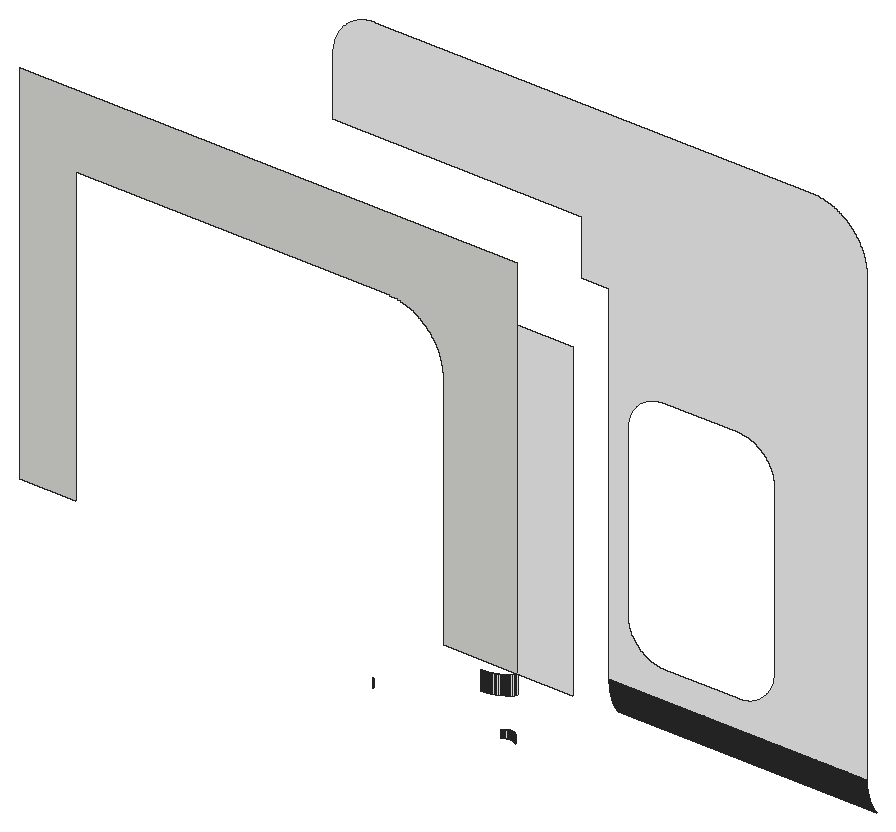
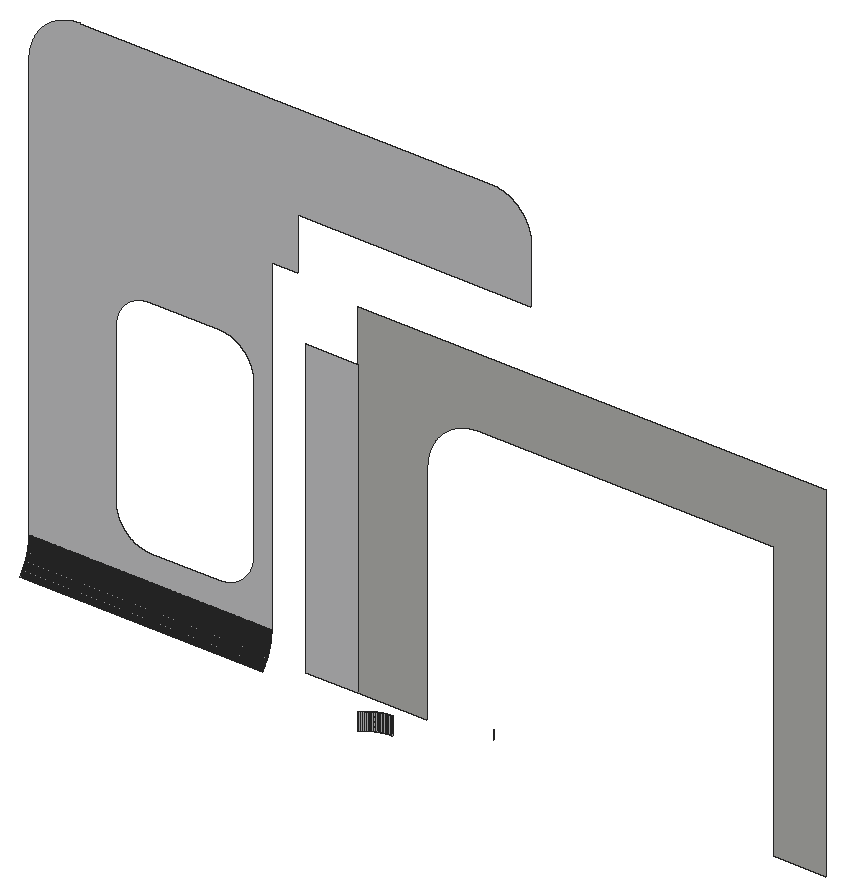
# SketchUp Ruby script. Lengths in inches.
U = 1.inch
M = Sketchup.active_model
def pt(a) = Geom::Point3d.new(a.map { |v| v * U })
def face(e, loops, mat)
  f = e.add_face(loops[0].map { |a| pt(a) })
  loops[1..].each { |l| e.add_face(l.map { |a| pt(a) }).erase! }
  f.material = f.back_material = mat if mat
  f
end
# faces: each face lists its corners as indices into pts; further lists are holes
def faces(e, pts, list, mat = nil) = list.each { |f| face(e, (f[0].is_a?(Array) ? f : [f]).map { |l| l.map { |i| pts[i] } }, mat) }
# xy, xz, yz: faces in a plane at the given z, y or x. An outline is a flat list of corners, or four numbers for a rectangle; further outlines are holes
def ring(l) = l.size == 4 ? [[l[0], l[1]], [l[2], l[1]], [l[2], l[3]], [l[0], l[3]]] : l.each_slice(2).to_a
def flat(e, list, mat, &to3) = list.each { |f| face(e, (f[0].is_a?(Array) ? f : [f]).map { |l| ring(l).map { |u, v| to3.(u, v) } }, mat) }
def xy(e, z, list, mat = nil) = flat(e, list, mat) { |x, y| [x, y, z] }
def xz(e, y, list, mat = nil) = flat(e, list, mat) { |x, z| [x, y, z] }
def yz(e, x, list, mat = nil) = flat(e, list, mat) { |y, z| [x, y, z] }
def lines(e, pts, list) = list.each { |a, b| e.add_line(pt(pts[a]), pt(pts[b])) }
# prism: a flat outline (further loops are holes) pulled along v
def prism(e, loops, v, mat = nil)
  f = face(e, loops, mat); d = Geom::Vector3d.new(v.map { |x| x * U })
  f.pushpull(f.normal.samedirection?(d) ? d.length : -d.length)
end
def box(e, o, s, mat = nil) = prism(e, [[o, [o[0] + s[0], o[1], o[2]], [o[0] + s[0], o[1] + s[1], o[2]], [o[0], o[1] + s[1], o[2]]]], [0, 0, s[2]], mat)
def at(x, y, z, deg = 0) = Geom::Transformation.translation(pt([x, y, z])) * Geom::Transformation.rotation(ORIGIN, Z_AXIS, deg.degrees)
def axes(o, x, y, z) = Geom::Transformation.new([*x, 0, *y, 0, *z, 0, *pt(o).to_a, 1])
def part(name) = M.definitions.add(name)
# library, detail: a bought-in or finely detailed component or shape, given as its bounding box
def library(name, o, s) = part(name).tap { |d| box(d.entities, o, s) }
def detail(e, o, s) = box(e.add_group.entities, o, s)
def put(e, d, t, mat = nil) = e.add_instance(d, t).tap { |i| i.material = mat if mat }
def group(e, t, mat = nil) = e.add_group.tap { |g| g.transformation = t; g.material = mat if mat }.entities
root = M.entities
M.materials.add("[Quartz Light Grey]").color = [251, 251, 252]
xz(root,256,[[207.84,117,207.92,119.5],[207.92,117,208,119.5],[208,117,208.08,119.5],[208.08,117,208.16,119.5]],"[Quartz Light Grey]")
xz(root,271,[[36,126,54,126,54,222,156.4,222,156.61,221.99,157.21,221.96,157.41,221.94,157.61,221.93,157.81,221.91,158.02,221.89,158.22,221.86,158.42,221.84,159.02,221.75,159.21,221.71,160.01,221.55,160.2,221.5,160.4,221.45,160.59,221.4,160.79,221.35,160.98,221.3,161.18,221.24,161.37,221.18,161.5625,221.12,161.75,221.06,161.95,220.99,162.14,220.92,162.32,220.85,162.7,220.71,162.89,220.63,163.07,220.55,163.26,220.47,163.44,220.39,163.63,220.3,163.81,220.22,164.35,219.95,164.71,219.75,164.88,219.66,165.06,219.55,165.4,219.35,165.58,219.24,165.92,219.02,166.08,218.91,166.25,218.8,166.42,218.68,166.58,218.5625,166.74,218.44,166.9,218.32,167.0625,218.2,167.22,218.07,167.38,217.95,167.54,217.82,167.69,217.6875,167.84,217.56,167.99,217.42,168.14,217.29,168.29,217.15,168.4375,217.01,168.58,216.87,168.73,216.73,168.87,216.58,169.01,216.4375,169.15,216.29,169.29,216.14,169.42,215.99,169.56,215.84,169.6875,215.69,169.82,215.54,169.95,215.38,170.07,215.22,170.2,215.0625,170.32,214.9,170.44,214.74,170.5625,214.58,170.68,214.42,170.8,214.25,170.91,214.08,171.02,213.92,171.24,213.58,171.35,213.4,171.55,213.06,171.66,212.88,171.75,212.71,171.95,212.35,172.22,211.81,172.3,211.63,172.39,211.44,172.47,211.26,172.55,211.07,172.63,210.89,172.71,210.7,172.85,210.32,172.92,210.14,172.99,209.95,173.06,209.75,173.12,209.5625,173.18,209.37,173.24,209.18,173.3,208.98,173.35,208.79,173.4,208.59,173.45,208.4,173.5,208.2,173.55,208.01,173.71,207.21,173.75,207.02,173.84,206.42,173.86,206.22,173.89,206.02,173.91,205.81,173.93,205.61,173.94,205.41,173.96,205.21,173.99,204.61,174,204.4,174,126,198,126,198,246,36,246]])
xz(root,271,[[186,117,186.16,123],[186.16,117,186.3125,123],[198,126,216,228],[228,134.77,312,135],[[228,135,312,135,312,282.24,311.99,282.47,311.99,282.71,311.98,282.94,311.96,283.18,311.94,283.41,311.92,283.65,311.9,283.88,311.875,284.12,311.85,284.35,311.8125,284.58,311.78,284.82,311.7,285.28,311.65,285.51,311.61,285.74,311.56,285.97,311.5,286.2,311.45,286.43,311.39,286.66,311.32,286.89,311.26,287.11,311.19,287.34,311.12,287.5625,311.04,287.79,310.97,288.01,310.89,288.23,310.8,288.45,310.72,288.67,310.54,289.11,310.44,289.32,310.35,289.54,310.25,289.75,310.14,289.96,310.04,290.17,309.82,290.59,309.7,290.8,309.59,291,309.35,291.4,309.22,291.61,309.1,291.8,308.97,292,308.83,292.2,308.7,292.39,308.5625,292.58,308.42,292.77,308.28,292.96,308.14,293.14,307.99,293.33,307.84,293.51,307.6875,293.69,307.53,293.87,307.375,294.04,307.22,294.22,307.06,294.39,306.89,294.56,306.73,294.73,306.56,294.89,306.39,295.06,306.22,295.22,306.04,295.375,305.87,295.53,305.69,295.6875,305.51,295.84,305.33,295.99,305.14,296.14,304.96,296.28,304.77,296.42,304.58,296.5625,304.39,296.7,304.2,296.83,304,296.97,303.8,297.1,303.61,297.22,303.4,297.35,303,297.59,302.8,297.7,302.59,297.82,302.17,298.04,301.96,298.14,301.75,298.25,301.54,298.35,301.32,298.44,301.11,298.54,300.67,298.72,300.45,298.8,300.23,298.89,300.01,298.97,299.79,299.04,299.5625,299.12,299.34,299.19,299.11,299.26,298.89,299.32,298.66,299.39,298.43,299.45,298.2,299.5,297.97,299.56,297.74,299.61,297.51,299.65,297.28,299.7,296.82,299.78,296.58,299.8125,296.35,299.85,296.12,299.875,295.88,299.9,295.65,299.92,295.41,299.94,295.18,299.96,294.94,299.98,294.71,299.99,294.47,299.99,294.24,300,151.63,300,151.27,299.98,151.08,299.97,150.9,299.96,150.54,299.92,150.35,299.9,149.99,299.86,149.45,299.77,148.55,299.57,148.2,299.47,148.02,299.42,147.85,299.37,147.67,299.31,147.5,299.26,147.33,299.2,147.15,299.13,146.98,299.07,146.8125,299,146.64,298.93,146.47,298.86,146.31,298.79,146.14,298.71,145.97,298.64,145.81,298.56,145.64,298.47,145.48,298.39,145.16,298.21,145,298.125,144.84,298.03,144.69,297.9375,144.53,297.84,144.22,297.64,144.07,297.54,143.92,297.43,143.77,297.33,143.48,297.11,143.33,296.99,143.19,296.88,143.05,296.76,142.91,296.65,142.77,296.53,142.63,296.4,142.5,296.28,142.36,296.16,141.84,295.64,141.72,295.5,141.6,295.37,141.47,295.23,141.35,295.09,141.24,294.95,141.12,294.81,141.01,294.67,140.89,294.52,140.67,294.23,140.57,294.08,140.46,293.93,140.36,293.78,140.16,293.47,140.0625,293.31,139.97,293.16,139.875,293,139.79,292.84,139.61,292.52,139.53,292.36,139.44,292.19,139.36,292.03,139.29,291.86,139.21,291.69,139.14,291.53,139.07,291.36,139,291.1875,138.93,291.02,138.87,290.85,138.8,290.67,138.74,290.5,138.69,290.33,138.63,290.15,138.58,289.98,138.53,289.8,138.43,289.45,138.23,288.55,138.14,288.01,138.1,287.65,138.08,287.46,138.04,287.1,138.03,286.92,138.02,286.73,138,286.37,138,267,219,267,219,249,228,249],[245.84,144,245.6875,144.01,245.53,144.01,245.37,144.02,245.22,144.03,244.9,144.05,244.75,144.07,244.59,144.08,244.43,144.1,244.28,144.125,244.12,144.15,243.97,144.17,243.8125,144.2,243.66,144.23,243.51,144.26,243.35,144.3,243.2,144.33,243.05,144.37,242.89,144.41,242.74,144.45,242.59,144.5,242.44,144.54,241.99,144.69,241.85,144.74,241.55,144.86,241.41,144.91,241.26,144.98,240.98,145.1,240.83,145.17,240.41,145.38,240.27,145.46,240.14,145.53,240,145.61,239.86,145.6875,239.73,145.77,239.6,145.85,239.46,145.9375,239.33,146.02,239.07,146.2,238.95,146.29,238.82,146.39,238.7,146.48,238.57,146.58,238.45,146.68,238.33,146.77,238.09,146.98,237.97,147.08,237.85,147.1875,237.74,147.3,237.52,147.52,237.4,147.63,237.3,147.74,237.1875,147.86,237.08,147.97,236.98,148.09,236.77,148.33,236.67,148.45,236.58,148.57,236.48,148.7,236.39,148.82,236.29,148.95,236.2,149.07,236.02,149.33,235.9375,149.47,235.85,149.6,235.77,149.73,235.6875,149.87,235.61,150,235.53,150.14,235.45,150.27,235.17,150.83,235.1,150.98,235.04,151.12,234.97,151.26,234.91,151.41,234.85,151.55,234.8,151.7,234.74,151.85,234.6875,151.99,234.64,152.14,234.49,152.59,234.41,152.89,234.37,153.05,234.33,153.2,234.3,153.35,234.26,153.51,234.23,153.66,234.2,153.8125,234.17,153.97,234.15,154.12,234.125,154.28,234.1,154.43,234.08,154.59,234.07,154.75,234.05,154.9,234.03,155.22,234.02,155.37,234.01,155.53,234,155.6875,234,210.3125,234.01,210.47,234.02,210.63,234.03,210.78,234.05,211.1,234.07,211.25,234.08,211.41,234.1,211.57,234.125,211.72,234.15,211.88,234.17,212.03,234.2,212.1875,234.23,212.34,234.26,212.49,234.3,212.65,234.33,212.8,234.37,212.95,234.41,213.11,234.49,213.41,234.64,213.86,234.6875,214.01,234.74,214.15,234.8,214.3,234.85,214.45,234.91,214.59,234.97,214.74,235.04,214.88,235.1,215.02,235.17,215.17,235.45,215.73,235.53,215.86,235.61,216,235.6875,216.14,235.77,216.27,235.85,216.4,235.9375,216.54,236.02,216.67,236.2,216.93,236.29,217.05,236.38,217.18,236.48,217.31,236.58,217.43,236.67,217.55,236.77,217.67,236.98,217.91,237.08,218.03,237.1875,218.15,237.3,218.26,237.4,218.375,237.51,218.49,237.625,218.6,237.74,218.7,237.85,218.8125,237.97,218.92,238.09,219.02,238.33,219.23,238.45,219.33,238.57,219.42,238.69,219.52,238.82,219.62,238.95,219.71,239.07,219.8,239.33,219.98,239.46,220.0625,239.6,220.15,239.73,220.23,239.86,220.3125,240,220.39,240.14,220.47,240.27,220.55,240.83,220.83,240.98,220.9,241.12,220.96,241.26,221.03,241.41,221.09,241.55,221.15,241.7,221.2,241.85,221.26,241.99,221.3125,242.14,221.36,242.59,221.51,242.89,221.59,243.05,221.63,243.2,221.67,243.35,221.7,243.51,221.74,243.66,221.77,243.8125,221.8,243.97,221.83,244.12,221.85,244.28,221.875,244.43,221.9,244.59,221.92,244.75,221.93,244.9,221.95,245.22,221.97,245.37,221.98,245.53,221.99,245.6875,222,270.3125,222,270.47,221.99,270.63,221.98,270.78,221.97,271.1,221.95,271.25,221.93,271.41,221.92,271.57,221.9,271.72,221.875,271.88,221.85,272.03,221.83,272.1875,221.8,272.34,221.77,272.49,221.74,272.65,221.7,272.8,221.67,272.95,221.63,273.11,221.59,273.41,221.51,273.86,221.36,274.01,221.3125,274.15,221.26,274.3,221.2,274.45,221.15,274.59,221.09,274.74,221.03,274.88,220.96,275.02,220.9,275.17,220.83,275.73,220.55,275.86,220.47,276,220.39,276.14,220.3125,276.27,220.23,276.4,220.15,276.54,220.0625,276.67,219.98,276.93,219.8,277.05,219.71,277.18,219.62,277.31,219.52,277.43,219.42,277.55,219.33,277.67,219.23,277.91,219.02,278.03,218.92,278.15,218.8125,278.26,218.7,278.375,218.6,278.49,218.49,278.6,218.375,278.7,218.26,278.8125,218.15,278.92,218.03,279.02,217.91,279.23,217.67,279.33,217.55,279.42,217.43,279.52,217.31,279.62,217.18,279.71,217.05,279.8,216.93,279.98,216.67,280.0625,216.54,280.15,216.4,280.23,216.27,280.3125,216.14,280.39,216,280.47,215.86,280.55,215.73,280.83,215.17,280.9,215.02,280.96,214.88,281.03,214.74,281.09,214.59,281.15,214.45,281.2,214.3,281.26,214.15,281.3125,214.01,281.36,213.86,281.51,213.41,281.59,213.11,281.63,212.95,281.67,212.8,281.7,212.65,281.74,212.49,281.77,212.34,281.8,212.1875,281.83,212.03,281.85,211.88,281.875,211.72,281.9,211.57,281.92,211.41,281.93,211.25,281.95,211.1,281.97,210.78,281.98,210.63,281.99,210.47,282,210.3125,282,155.6875,281.99,155.53,281.98,155.37,281.97,155.22,281.95,154.9,281.93,154.75,281.92,154.59,281.9,154.43,281.875,154.28,281.85,154.12,281.83,153.97,281.8,153.8125,281.77,153.66,281.74,153.51,281.7,153.35,281.67,153.2,281.63,153.05,281.59,152.89,281.51,152.59,281.36,152.14,281.3125,151.99,281.26,151.85,281.2,151.7,281.15,151.55,281.09,151.41,281.03,151.26,280.96,151.12,280.9,150.98,280.83,150.83,280.55,150.27,280.47,150.14,280.39,150,280.3125,149.87,280.23,149.73,280.15,149.6,280.0625,149.47,279.98,149.33,279.8,149.07,279.71,148.95,279.61,148.82,279.52,148.7,279.42,148.57,279.33,148.45,279.23,148.33,279.02,148.09,278.92,147.97,278.8125,147.86,278.7,147.74,278.6,147.63,278.48,147.52,278.26,147.3,278.15,147.1875,278.03,147.08,277.91,146.98,277.67,146.77,277.55,146.68,277.43,146.58,277.3,146.48,277.18,146.39,277.05,146.29,276.93,146.2,276.67,146.02,276.54,145.9375,276.4,145.85,276.27,145.77,276.14,145.6875,276,145.61,275.86,145.53,275.73,145.46,275.59,145.38,275.17,145.17,275.02,145.1,274.74,144.98,274.59,144.91,274.45,144.86,274.15,144.74,274.01,144.69,273.56,144.54,273.41,144.5,273.26,144.45,273.11,144.41,272.95,144.37,272.8,144.33,272.65,144.3,272.49,144.26,272.34,144.23,272.1875,144.2,272.03,144.17,271.88,144.15,271.72,144.125,271.57,144.1,271.41,144.08,271.25,144.07,271.1,144.05,270.78,144.03,270.63,144.02,270.47,144.01,270.3125,144.01,270.16,144]]],"[Quartz Light Grey]")
xz(root,271.01,[[228,134.29,312,134.53]],"[Quartz Light Grey]")
p = [[164,254.89,117],[164.05,254.83,117],[164.05,254.83,119.5],[164,254.89,119.5],[163.9,255.01,117],[163.95,254.95,117],
  [163.95,254.95,119.5],[163.9,255.01,119.5],[205.67,254.89,117],[205.72,254.95,117],[205.72,254.95,119.5],[205.67,254.89,119.5],
  [205.77,255.01,117],[205.77,255.01,119.5],[210.23,255.01,117],[210.28,254.95,117],[210.28,254.95,119.5],[210.23,255.01,119.5],
  [210.33,254.89,117],[210.33,254.89,119.5],[163.84,255.07,117],[163.84,255.07,119.5],[205.82,255.07,117],[205.82,255.07,119.5],
  [210.18,255.07,117],[210.18,255.07,119.5],[163.73,255.18,117],[163.79,255.12,117],[163.79,255.12,119.5],[163.73,255.18,119.5],
  [205.88,255.12,117],[205.88,255.12,119.5],[205.93,255.18,117],[205.93,255.18,119.5],[210.07,255.18,117],[210.12,255.12,117],
  [210.12,255.12,119.5],[210.07,255.18,119.5],[163.62,255.28,117],[163.67,255.23,117],[163.67,255.23,119.5],[163.62,255.28,119.5],
  [205.99,255.23,117],[205.99,255.23,119.5],[206.05,255.28,117],[206.05,255.28,119.5],[209.95,255.28,117],[210.01,255.23,117],
  [210.01,255.23,119.5],[209.95,255.28,119.5],[163.49,255.38,117],[163.55,255.33,117],[163.55,255.33,119.5],[163.49,255.38,119.5],
  [206.11,255.33,117],[206.11,255.33,119.5],[206.17,255.38,117],[206.17,255.38,119.5],[209.83,255.38,117],[209.89,255.33,117],
  [209.89,255.33,119.5],[209.83,255.38,119.5],[163.37,255.47,117],[163.43,255.43,117],[163.43,255.43,119.5],[163.37,255.47,119.5],
  [206.24,255.43,117],[206.24,255.43,119.5],[206.3,255.47,117],[206.3,255.47,119.5],[209.7,255.47,117],[209.76,255.43,117],
  [209.76,255.43,119.5],[209.7,255.47,119.5],[163.3,255.52,117],[163.3,255.52,119.5],[206.37,255.52,117],[206.37,255.52,119.5],
  [206.43,255.56,117],[206.43,255.56,119.5],[209.57,255.56,117],[209.63,255.52,117],[209.63,255.52,119.5],[209.57,255.56,119.5],
  [206.5,255.6,117],[206.5,255.6,119.5],[206.57,255.64,117],[206.57,255.64,119.5],[206.64,255.67,117],[206.64,255.67,119.5],
  [209.36,255.67,117],[209.43,255.64,117],[209.43,255.64,119.5],[209.36,255.67,119.5],[209.5,255.6,117],[209.5,255.6,119.5],
  [206.71,255.71,117],[206.71,255.71,119.5],[206.78,255.74,117],[206.78,255.74,119.5],[206.85,255.77,117],[206.85,255.77,119.5],
  [209.15,255.77,117],[209.22,255.74,117],[209.22,255.74,119.5],[209.15,255.77,119.5],[209.29,255.71,117],[209.29,255.71,119.5],
  [206.92,255.8,117],[206.92,255.8,119.5],[207,255.83,117],[207,255.83,119.5],[207.07,255.85,117],[207.07,255.85,119.5],
  [208.93,255.85,117],[209,255.83,117],[209,255.83,119.5],[208.93,255.85,119.5],[209.08,255.8,117],[209.08,255.8,119.5],
  [207.15,255.875,117],[207.15,255.875,119.5],[207.22,255.9,117],[207.22,255.9,119.5],[207.3,255.92,117],[207.3,255.92,119.5],
  [207.375,255.93,117],[207.375,255.93,119.5],[207.45,255.95,117],[207.45,255.95,119.5],[207.53,255.96,117],[207.53,255.96,119.5],
  [208.47,255.96,117],[208.55,255.95,117],[208.55,255.95,119.5],[208.47,255.96,119.5],[208.625,255.93,117],[208.625,255.93,119.5],
  [208.7,255.92,117],[208.7,255.92,119.5],[208.78,255.9,117],[208.78,255.9,119.5],[208.85,255.875,117],[208.85,255.875,119.5],
  [207.61,255.97,117],[207.61,255.97,119.5],[207.6875,255.98,117],[207.6875,255.98,119.5],[207.76,255.99,117],[207.76,255.99,119.5],
  [207.84,256,117],[207.84,256,119.5],[208.16,256,117],[208.24,255.99,117],[208.24,255.99,119.5],[208.16,256,119.5],
  [208.3125,255.98,117],[208.3125,255.98,119.5],[208.39,255.97,117],[208.39,255.97,119.5],[186.47,271.01,117],[186.3125,271,117],
  [186.3125,271,123],[186.47,271.01,123],[186.63,271.02,117],[186.63,271.02,123],[186.78,271.03,117],[186.78,271.03,123],
  [186.94,271.04,117],[186.94,271.04,123],[187.1,271.05,117],[187.1,271.05,123],[187.25,271.07,117],[187.25,271.07,123],
  [187.41,271.08,117],[187.41,271.08,123],[187.57,271.1,117],[187.57,271.1,123],[187.72,271.125,117],[187.72,271.125,123],
  [187.88,271.15,117],[187.88,271.15,123],[188.03,271.17,117],[188.03,271.17,123],[188.1875,271.2,117],[188.1875,271.2,123],
  [188.34,271.23,117],[188.34,271.23,123],[188.49,271.26,117],[188.49,271.26,123],[188.65,271.3,117],[188.65,271.3,123],
  [188.8,271.33,117],[188.8,271.33,123],[188.95,271.37,117],[188.95,271.37,123],[189.11,271.41,117],[189.11,271.41,123],
  [189.26,271.45,117],[189.26,271.45,123],[189.41,271.49,117],[189.41,271.49,123],[189.56,271.54,117],[189.56,271.54,123],
  [189.71,271.59,117],[189.71,271.59,123],[189.86,271.64,117],[189.86,271.64,123],[190.01,271.6875,117],[190.01,271.6875,123],
  [190.15,271.74,117],[190.15,271.74,123],[190.3,271.8,117],[190.3,271.8,123],[190.45,271.85,117],[190.45,271.85,123],
  [190.59,271.91,117],[190.59,271.91,123],[190.74,271.97,117],[190.74,271.97,123],[190.88,272.04,117],[190.88,272.04,123],
  [191.02,272.1,117],[191.02,272.1,123],[191.17,272.17,117],[191.17,272.17,123],[191.31,272.24,117],[191.31,272.24,123],
  [191.45,272.31,117],[191.45,272.31,123],[191.59,272.38,117],[191.59,272.38,123],[191.73,272.45,117],[191.73,272.45,123],
  [191.86,272.53,117],[191.86,272.53,123],[192,272.61,117],[192,272.61,123],[192.14,272.6875,117],[192.14,272.6875,123],
  [192.27,272.77,117],[192.27,272.77,123],[192.4,272.85,117],[192.4,272.85,123],[192.54,272.9375,117],[192.54,272.9375,123],
  [192.67,273.02,117],[192.67,273.02,123],[192.8,273.11,117],[192.8,273.11,123],[192.93,273.2,117],[192.93,273.2,123],
  [193.05,273.29,117],[193.05,273.29,123],[193.18,273.38,117],[193.18,273.38,123],[193.31,273.48,117],[193.31,273.48,123],
  [193.43,273.58,117],[193.43,273.58,123],[193.55,273.67,117],[193.55,273.67,123],[193.67,273.77,117],[193.67,273.77,123],
  [193.79,273.875,117],[193.79,273.875,123],[193.91,273.98,117],[193.91,273.98,123],[194.03,274.08,117],[194.03,274.08,123],
  [194.15,274.1875,117],[194.15,274.1875,123],[194.26,274.3,117],[194.26,274.3,123],[194.375,274.4,117],[194.375,274.4,123],
  [194.49,274.51,117],[194.49,274.51,123],[194.6,274.625,117],[194.6,274.625,123],[194.7,274.74,117],[194.7,274.74,123],
  [194.8125,274.85,117],[194.8125,274.85,123],[194.92,274.97,117],[194.92,274.97,123],[312,274.86,123.86],[312,274.72,124.04],
  [228,274.72,124.04],[228,274.86,123.86],[312,274.58,124.23],[228,274.58,124.23],[312,274.4375,124.42],[228,274.4375,124.42],
  [312,274.3,124.61],[228,274.3,124.61],[312,274.17,124.81],[228,274.17,124.81],[312,274.03,125],[228,274.03,125],
  [312,273.9,125.2],[228,273.9,125.2],[312,273.78,125.4],[228,273.78,125.4],[312,273.65,125.6],[228,273.65,125.6],
  [312,273.53,125.8],[228,273.53,125.8],[312,273.41,126],[228,273.41,126],[312,273.3,126.21],[228,273.3,126.21],
  [312,273.18,126.41],[228,273.18,126.41],[312,273.07,126.62],[228,273.07,126.62],[312,272.96,126.83],[228,272.96,126.83],
  [312,272.86,127.04],[228,272.86,127.04],[312,272.75,127.25],[228,272.75,127.25],[312,272.65,127.46],[228,272.65,127.46],
  [312,272.56,127.68],[228,272.56,127.68],[312,272.46,127.9],[228,272.46,127.9],[312,272.37,128.11],[228,272.37,128.11],
  [312,272.28,128.33],[228,272.28,128.33],[312,272.2,128.55],[228,272.2,128.55],[312,272.11,128.77],[228,272.11,128.77],
  [312,272.03,128.99],[228,272.03,128.99],[312,271.96,129.22],[228,271.96,129.22],[312,271.88,129.4375],[228,271.88,129.4375],
  [312,271.81,129.66],[228,271.81,129.66],[312,271.74,129.89],[228,271.74,129.89],[312,271.68,130.12],[228,271.68,130.12],
  [312,271.61,130.34],[228,271.61,130.34],[312,271.55,130.57],[228,271.55,130.57],[312,271.5,130.8],[228,271.5,130.8],
  [312,271.44,131.03],[228,271.44,131.03],[312,271.39,131.26],[228,271.39,131.26],[312,271.35,131.49],[228,271.35,131.49],
  [312,271.3,131.72],[228,271.3,131.72],[312,271.26,131.95],[228,271.26,131.95],[312,271.22,132.19],[228,271.22,132.19],
  [312,271.1875,132.42],[228,271.1875,132.42],[312,271.15,132.65],[228,271.15,132.65],[312,271.125,132.89],[228,271.125,132.89],
  [312,271.1,133.12],[228,271.1,133.12],[312,271.08,133.35],[228,271.08,133.35],[312,271.06,133.59],[228,271.06,133.59],
  [312,271.04,133.82],[228,271.04,133.82],[312,271.02,134.06],[228,271.02,134.06],[312,271.01,134.29],[228,271.01,134.29],
  [312,271.01,134.53],[312,271,134.77],[228,271,134.77],[228,271.01,134.53]]
faces(root,p,[[0,1,2,3],[4,5,6,7],[5,0,3,6],[8,9,10,11],[9,12,13,10],[14,15,16,17],[15,18,19,16],[20,4,7,21],
  [12,22,23,13],[24,14,17,25],[26,27,28,29],[27,20,21,28],[22,30,31,23],[30,32,33,31],[34,35,36,37],[35,24,25,36],
  [38,39,40,41],[39,26,29,40],[32,42,43,33],[42,44,45,43],[46,47,48,49],[47,34,37,48],[50,51,52,53],[51,38,41,52],
  [44,54,55,45],[54,56,57,55],[58,59,60,61],[59,46,49,60],[62,63,64,65],[63,50,53,64],[56,66,67,57],[66,68,69,67],
  [70,71,72,73],[71,58,61,72],[74,62,65,75],[68,76,77,69],[76,78,79,77],[80,81,82,83],[81,70,73,82],[78,84,85,79],
  [84,86,87,85],[86,88,89,87],[90,91,92,93],[91,94,95,92],[94,80,83,95],[88,96,97,89],[96,98,99,97],[98,100,101,99],
  [102,103,104,105],[103,106,107,104],[106,90,93,107],[100,108,109,101],[108,110,111,109],[110,112,113,111],[114,115,116,117],[115,118,119,116],
  [118,102,105,119],[112,120,121,113],[120,122,123,121],[122,124,125,123],[124,126,127,125],[126,128,129,127],[128,130,131,129],[132,133,134,135],
  [133,136,137,134],[136,138,139,137],[138,140,141,139],[140,142,143,141],[142,114,117,143],[130,144,145,131],[144,146,147,145],[146,148,149,147],
  [148,150,151,149],[152,153,154,155],[153,156,157,154],[156,158,159,157],[158,132,135,159],[160,161,162,163],[164,160,163,165],[166,164,165,167],
  [168,166,167,169],[170,168,169,171],[172,170,171,173],[174,172,173,175],[176,174,175,177],[178,176,177,179],[180,178,179,181],[182,180,181,183],
  [184,182,183,185],[186,184,185,187],[188,186,187,189],[190,188,189,191],[192,190,191,193],[194,192,193,195],[196,194,195,197],[198,196,197,199],
  [200,198,199,201],[202,200,201,203],[204,202,203,205],[206,204,205,207],[208,206,207,209],[210,208,209,211],[212,210,211,213],[214,212,213,215],
  [216,214,215,217],[218,216,217,219],[220,218,219,221],[222,220,221,223],[224,222,223,225],[226,224,225,227],[228,226,227,229],[230,228,229,231],
  [232,230,231,233],[234,232,233,235],[236,234,235,237],[238,236,237,239],[240,238,239,241],[242,240,241,243],[244,242,243,245],[246,244,245,247],
  [248,246,247,249],[250,248,249,251],[252,250,251,253],[254,252,253,255],[256,254,255,257],[258,256,257,259],[260,258,259,261],[262,260,261,263],
  [264,262,263,265],[266,264,265,267],[268,266,267,269],[270,268,269,271],[272,270,271,273],[274,272,273,275],[276,274,275,277],[278,276,277,279],
  [280,278,279,281],[282,280,281,283],[284,282,283,285],[286,287,288,289],[287,290,291,288],[290,292,293,291],[292,294,295,293],[294,296,297,295],
  [296,298,299,297],[298,300,301,299],[300,302,303,301],[302,304,305,303],[304,306,307,305],[306,308,309,307],[308,310,311,309],[310,312,313,311],
  [312,314,315,313],[314,316,317,315],[316,318,319,317],[318,320,321,319],[320,322,323,321],[322,324,325,323],[324,326,327,325],[326,328,329,327],
  [328,330,331,329],[330,332,333,331],[332,334,335,333],[334,336,337,335],[336,338,339,337],[338,340,341,339],[340,342,343,341],[342,344,345,343],
  [344,346,347,345],[346,348,349,347],[348,350,351,349],[350,352,353,351],[352,354,355,353],[354,356,357,355],[356,358,359,357],[358,360,361,359],
  [360,362,363,361],[362,364,365,363],[364,366,367,365],[366,368,369,367],[368,370,371,369],[370,372,373,371],[372,374,375,373],[374,376,377,375],
  [376,378,379,377],[378,380,381,379],[380,382,383,381],[384,385,386,387]],"[Quartz Light Grey]")
